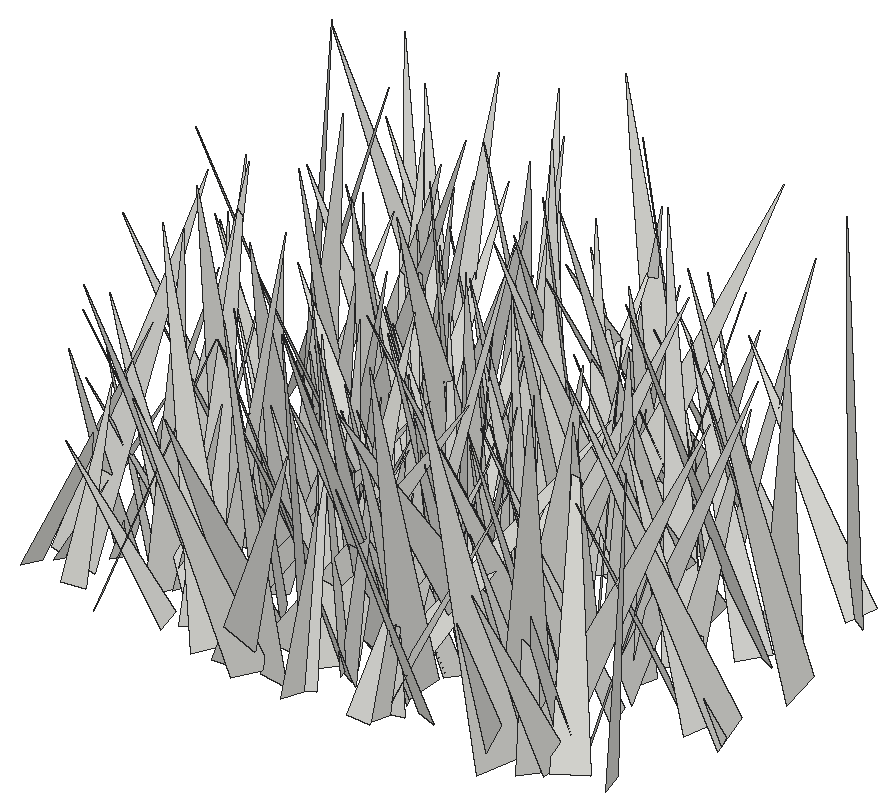
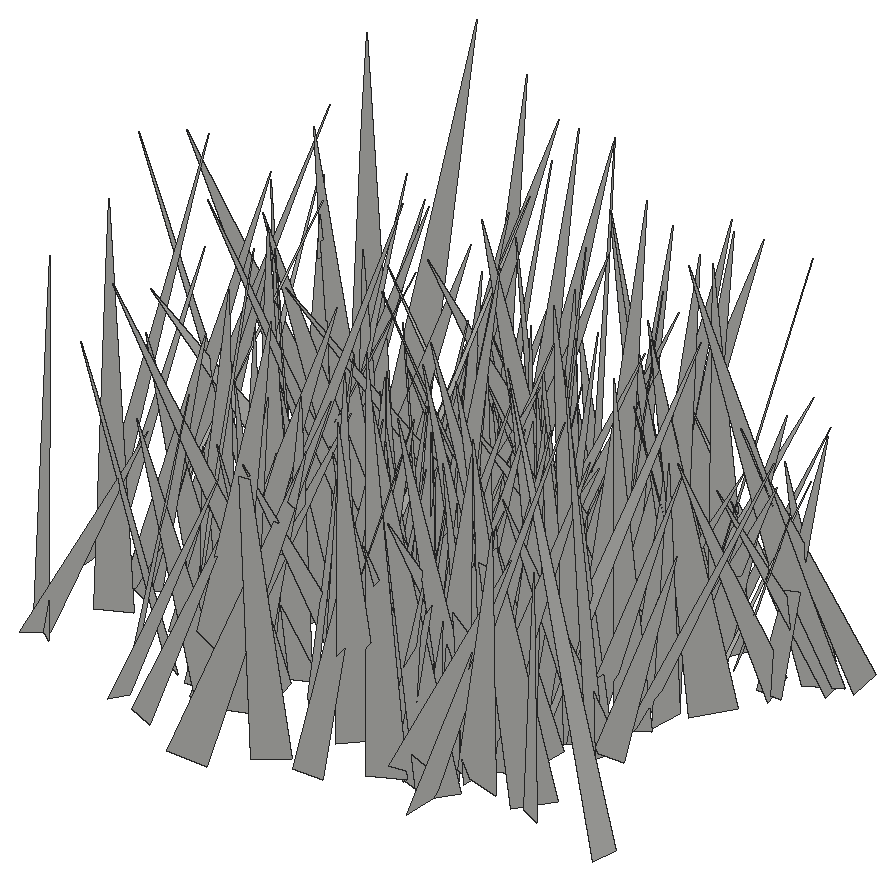
# SketchUp Ruby script. Lengths in inches.
U = 1.inch
M = Sketchup.active_model
def pt(a) = Geom::Point3d.new(a.map { |v| v * U })
def face(e, loops, mat)
  f = e.add_face(loops[0].map { |a| pt(a) })
  loops[1..].each { |l| e.add_face(l.map { |a| pt(a) }).erase! }
  f.material = f.back_material = mat if mat
  f
end
# faces: each face lists its corners as indices into pts; further lists are holes
def faces(e, pts, list, mat = nil) = list.each { |f| face(e, (f[0].is_a?(Array) ? f : [f]).map { |l| l.map { |i| pts[i] } }, mat) }
# xy, xz, yz: faces in a plane at the given z, y or x. An outline is a flat list of corners, or four numbers for a rectangle; further outlines are holes
def ring(l) = l.size == 4 ? [[l[0], l[1]], [l[2], l[1]], [l[2], l[3]], [l[0], l[3]]] : l.each_slice(2).to_a
def flat(e, list, mat, &to3) = list.each { |f| face(e, (f[0].is_a?(Array) ? f : [f]).map { |l| ring(l).map { |u, v| to3.(u, v) } }, mat) }
def xy(e, z, list, mat = nil) = flat(e, list, mat) { |x, y| [x, y, z] }
def xz(e, y, list, mat = nil) = flat(e, list, mat) { |x, z| [x, y, z] }
def yz(e, x, list, mat = nil) = flat(e, list, mat) { |y, z| [x, y, z] }
def lines(e, pts, list) = list.each { |a, b| e.add_line(pt(pts[a]), pt(pts[b])) }
# prism: a flat outline (further loops are holes) pulled along v
def prism(e, loops, v, mat = nil)
  f = face(e, loops, mat); d = Geom::Vector3d.new(v.map { |x| x * U })
  f.pushpull(f.normal.samedirection?(d) ? d.length : -d.length)
end
def box(e, o, s, mat = nil) = prism(e, [[o, [o[0] + s[0], o[1], o[2]], [o[0] + s[0], o[1] + s[1], o[2]], [o[0], o[1] + s[1], o[2]]]], [0, 0, s[2]], mat)
def at(x, y, z, deg = 0) = Geom::Transformation.translation(pt([x, y, z])) * Geom::Transformation.rotation(ORIGIN, Z_AXIS, deg.degrees)
def axes(o, x, y, z) = Geom::Transformation.new([*x, 0, *y, 0, *z, 0, *pt(o).to_a, 1])
def part(name) = M.definitions.add(name)
# library, detail: a bought-in or finely detailed component or shape, given as its bounding box
def library(name, o, s) = part(name).tap { |d| box(d.entities, o, s) }
def detail(e, o, s) = box(e.add_group.entities, o, s)
def put(e, d, t, mat = nil) = e.add_instance(d, t).tap { |i| i.material = mat if mat }
def group(e, t, mat = nil) = e.add_group.tap { |g| g.transformation = t; g.material = mat if mat }.entities
root = M.entities
c1 = part("fur_instance\#9")
p = [[0.8125,0,1.79],[0.67,-0.02,1.48],[0,-0.11,0],[0,0.11,0]]
faces(c1.entities,p,[[0,1,2,3]])
put(root,c1,axes([490.59,5.4,-21.86],[2.87814,-5.28951,1.31735],[-4.95416,-3.15966,-1.86304],[-2.27391,0.18887,5.72641]))
put(root,c1,axes([500.76,5.73,-21.86],[6.46231,-4.31648,2.52967],[-3.92803,-6.93665,-1.8017],[-3.09867,-0.20881,7.55958]))
put(root,c1,axes([489.84,5.36,-21.86],[2.89446,-5.47209,0.08006],[-5.31049,-2.7865,1.53693],[1.32243,0.78724,5.99662]))
put(root,c1,axes([500.48,6.03,-21.86],[4.1039,-1.37964,0.4984],[-1.03776,-3.77714,-1.91052],[-1.03675,-1.68037,3.88527]))
put(root,c1,axes([489.15,7.79,-21.86],[5.11337,-4.37567,0.02712],[-4.08728,-4.79107,-2.37351],[-1.56248,-1.78687,6.29758]))
put(root,c1,axes([502.23,6.75,-21.86],[4.14247,-2.36814,0.94959],[-1.79033,-3.98803,-2.13546],[-1.81783,-1.46881,4.26707]))
put(root,c1,axes([492.5625,5.1,-21.86],[3.76138,-1.24538,0.93866],[-1.27843,-3.86595,-0.00634],[-0.89313,0.28885,3.96218]))
put(root,c1,axes([486.36,6.41,-21.86],[-3.93279,-0.23592,0.50656],[-0.05149,3.7386,1.34138],[0.55643,-1.32147,3.70448]))
put(root,c1,axes([491.49,5.47,-21.86],[1.25077,5.74635,3.18749],[6.40163,-1.79789,0.7292],[-1.48314,-2.91412,5.83551]))
put(root,c1,axes([491.71,6.95,-21.86],[6.5233,2.37968,3.04495],[3.30026,-6.53866,-1.96019],[-2.01069,-3.01183,6.66138]))
put(root,c1,axes([495.69,7.7,-21.86],[7.48346,-2.4752,1.75576],[-1.96533,-7.51292,-2.21472],[-2.31232,-1.62508,7.56464]))
put(root,c1,axes([496.91,6.61,-21.86],[-1.89303,-4.40404,0.51291],[-4.43222,1.86471,-0.34716],[-0.11875,0.60786,4.78107]))
put(root,c1,axes([495.44,7.87,-21.86],[-5.97447,-2.65496,2.2585],[-2.10106,6.3191,1.8704],[2.78122,-0.92951,6.26456]))
put(root,c1,axes([499.77,8.2,-21.86],[5.80631,-5.6916,0.53269],[-5.68589,-5.82856,-0.29992],[-0.59055,0.15799,8.12513]))
put(root,c1,axes([495.26,5.15,-21.86],[-0.85161,3.55792,0.87868],[3.50079,1.05663,-0.88551],[1.08413,-0.61714,3.54963]))
put(root,c1,axes([495.77,5.74,-21.86],[3.9323,-0.29865,1.47953],[-0.48436,-4.16008,0.44758],[-1.42954,0.58799,3.91814]))
put(root,c1,axes([488.64,5.97,-21.86],[5.34271,-3.44394,4.19103],[-3.85612,-6.54857,-0.46545],[-3.8152,1.796,6.33945]))
put(root,c1,axes([492.67,5.54,-21.86],[-2.63101,2.88231,1.12737],[2.88894,2.81797,-0.46255],[1.11028,-0.50218,3.87505]))
put(root,c1,axes([493.65,9.14,-21.86],[-1.56855,-7.63886,0.47282],[-7.63369,1.59619,0.46371],[0.55001,0.36889,7.78444]))
put(root,c1,axes([493.09,9.02,-21.86],[-1.24529,-7.71146,0.7872],[-7.61167,1.36728,1.35282],[1.46589,0.54863,7.69333]))
put(root,c1,axes([495.97,6.11,-21.86],[-0.42673,3.51272,1.26133],[3.73148,0.37463,0.21911],[-0.0791,-1.27778,3.53176]))
put(root,c1,axes([485.99,8.94,-21.86],[-5.87667,-3.9224,1.1719],[-3.54254,5.90008,1.98324],[2.05159,-1.04767,6.78139]))
put(root,c1,axes([496.43,11.28,-21.86],[6.48177,-5.01878,0.45242],[-4.24735,-5.8379,-3.90962],[-2.71162,-2.85253,7.2053]))
put(root,c1,axes([482.5,6.33,-21.86],[1.50954,-3.07856,1.78204],[-3.55315,-1.39659,0.59714],[-0.16832,1.87187,3.37633]))
put(root,c1,axes([495.36,6.375,-21.86],[4.26257,2.91433,0.00484],[2.86478,-4.18851,-0.95515],[0.53516,-0.79116,5.0745]))
put(root,c1,axes([493.22,7.15,-21.86],[-4.07281,-4.5818,0.7427],[-4.55178,3.7491,-1.83244],[-0.90871,1.75604,5.85003]))
put(root,c1,axes([502.5,7.23,-21.86],[-2.82559,-5.19892,1.36333],[-5.31081,2.46391,-1.61114],[-0.82624,1.9421,5.69358]))
put(root,c1,axes([493.16,7.29,-21.86],[-2.2184,-4.85625,2.50772],[-5.03427,2.86928,1.10295],[2.1279,1.72546,5.22379]))
put(root,c1,axes([483.85,5.87,-21.86],[4.67763,2.46387,0.32375],[2.42875,-4.67875,0.51598],[-0.52599,0.30722,5.26162]))
put(root,c1,axes([488.33,6.51,-21.86],[3.51282,6.48869,2.15536],[6.79895,-3.57131,-0.32959],[-0.72316,-2.057,7.37118]))
put(root,c1,axes([494.02,9.8,-21.86],[0.91658,-6.09487,0.23316],[-5.96683,-0.94489,-1.24341],[-1.26442,0.04079,6.03668]))
put(root,c1,axes([504.33,6.97,-21.86],[-4.83531,-1.63891,2.39644],[-2.01972,5.24312,-0.48946],[2.08559,1.27782,5.08199]))
put(root,c1,axes([485.08,7.92,-21.86],[-5.61419,2.77509,3.47904],[3.15086,6.4338,-0.04739],[3.14276,-1.49299,6.26243]))
put(root,c1,axes([486.97,8.74,-21.86],[-3.76268,-4.24685,0.11424],[-4.17448,3.66755,-1.15295],[-0.78896,0.84846,5.55555]))
put(root,c1,axes([480.48,6.67,-21.86],[5.14686,-0.10254,0.48257],[-0.21946,-5.00543,1.27711],[-0.44184,1.29176,4.98695]))
put(root,c1,axes([482.52,9.11,-21.86],[-0.08561,-4.51883,0.61864],[-4.55746,0.06047,-0.18896],[-0.17898,0.62161,4.51569]))
put(root,c1,axes([492.46,7.47,-21.86],[-4.38445,3.57185,1.79964],[3.76738,4.58485,0.07863],[1.34299,-1.20052,5.65467]))
put(root,c1,axes([501.79,5.78,-21.86],[-6.16922,0.32467,1.04524],[-0.06119,5.87189,-2.18505],[1.09279,2.16166,5.77844]))
put(root,c1,axes([492.85,7.61,-21.86],[-6.07164,-2.28107,2.04855],[-2.55827,6.27412,-0.5961],[1.68971,1.3026,6.45854]))
put(root,c1,axes([491.02,9.64,-21.86],[-1.13114,-4.608,0.05517],[-4.59723,1.12439,-0.34274],[-0.31976,0.13515,4.73241]))
put(root,c1,axes([490.4,7.86,-21.86],[4.34126,2.62004,0.01209],[2.52851,-4.18338,-1.34808],[0.68659,-1.1602,4.88813]))
put(root,c1,axes([490.38,7.3125,-21.86],[4.70359,-4.43483,0.77561],[-4.1988,-3.91632,3.07011],[1.62462,2.71804,5.6891]))
put(root,c1,axes([502.88,6.61,-21.86],[-3.10471,5.12305,0.88051],[5.18598,3.12286,0.11631],[0.35573,-0.81381,5.98927]))
put(root,c1,axes([489.07,9.04,-21.86],[-4.89402,-3.33819,1.83703],[-3.30827,5.20635,0.64726],[1.89038,0.46913,5.88863]))
put(root,c1,axes([500.16,10.02,-21.86],[-3.94207,-4.94022,1.13908],[-4.81769,4.09962,1.10733],[1.57897,0.1748,6.2225]))
put(root,c1,axes([485.38,8.5,-21.86],[3.78435,-1.32179,0.68035],[-1.35222,-3.83372,0.07338],[-0.61764,0.29457,4.00787]))
put(root,c1,axes([492.36,7.69,-21.86],[-1.02594,6.32348,2.52203],[6.58274,1.57191,-1.26344],[1.73626,-2.22313,6.28034]))
put(root,c1,axes([491.15,9.28,-21.86],[1.24719,-3.91493,0.4967],[-3.8954,-1.13791,0.81231],[0.63182,0.71228,4.02769]))
put(root,c1,axes([492.39,9.25,-21.86],[-1.33091,-4.34516,1.37723],[-4.35803,1.6335,0.94222],[1.33595,0.99989,4.44566]))
put(root,c1,axes([485.41,8.57,-21.86],[0.69074,-4.72184,2.34998],[-4.89788,-1.45354,-1.48096],[-1.95676,1.97148,4.53648]))
put(root,c1,axes([481.08,7.53,-21.86],[4.0967,-0.1052,0.02727],[-0.10864,-3.93802,1.12914],[0.00278,1.12946,3.93942]))
put(root,c1,axes([486.375,8.03,-21.86],[-2.33068,3.85921,0.35584],[3.66264,2.05758,1.6744],[-1.26695,-1.15111,4.18592]))
put(root,c1,axes([481.46,7.63,-21.86],[0.24663,7.62872,2.41582],[7.70784,0.42293,-2.12242],[2.15005,-2.39126,7.33168]))
put(root,c1,axes([496.5,9.66,-21.86],[-2.38494,-6.16406,1.52656],[-6.35023,2.30898,-0.59758],[-0.0234,1.63919,6.58229]))
put(root,c1,axes([500.99,7.71,-21.86],[5.79439,-3.93356,1.43708],[-4.17619,-5.2444,2.48372],[0.31237,2.85246,6.54821]))
put(root,c1,axes([484.71,7.97,-21.86],[-3.84784,-1.19504,0.32807],[-1.23606,3.62421,-1.29571],[-0.08892,1.33363,3.81512]))
put(root,c1,axes([498.37,9.9,-21.86],[-3.36385,-0.86607,1.07357],[-0.51946,3.41676,1.12873],[1.27781,-0.89095,3.28504]))
put(root,c1,axes([495.2,9.57,-21.86],[-3.34237,-3.67886,0.49489],[-3.71061,3.29315,-0.58039],[-0.10119,0.75599,4.93646]))
put(root,c1,axes([484.01,10.37,-21.86],[-3.17916,-2.57933,0.00353],[-2.53731,3.12837,0.73174],[0.46373,-0.56605,4.02798]))
put(root,c1,axes([497.12,9.2,-21.86],[-3.3946,-3.12525,1.18102],[-3.29173,3.41661,-0.4203],[0.5714,1.11577,4.59499]))
put(root,c1,axes([498.01,11.3,-21.86],[2.24091,-5.47361,0.67385],[-5.23088,-2.33999,-1.61199],[-1.7471,-0.01469,5.69066]))
put(root,c1,axes([490.29,8.67,-21.86],[4.49912,0.07902,0.02983],[0.07502,-4.46879,0.52292],[-0.03881,0.52233,4.46932]))
put(root,c1,axes([490.03,10.12,-21.86],[1.8485,-3.49978,1.33816],[-3.45042,-2.17169,-0.91344],[-1.46071,0.70098,3.8511]))
put(root,c1,axes([502.19,12.9,-21.86],[-3.50557,-5.51536,0.11612],[-4.95597,3.20905,2.80393],[2.42302,-1.41579,5.90306]))
put(root,c1,axes([498.3,10.3125,-21.86],[2.2039,-6.87435,1.74953],[-7.02125,-1.85328,1.56272],[1.00974,2.1174,7.04782]))
put(root,c1,axes([495.91,9.36,-21.86],[-0.77186,4.35622,1.72795],[4.2436,-0.09339,2.13104],[-1.98854,-1.8902,3.87699]))
put(root,c1,axes([505.26,11.92,-21.86],[-7.42684,-1.75978,1.28146],[-1.36577,7.3143,2.12899],[1.69519,-1.81689,7.32954]))
put(root,c1,axes([501.73,10.57,-21.86],[-5.35424,-1.86738,0.02315],[-1.86377,5.3475,0.29345],[0.11847,-0.26947,5.66294]))
put(root,c1,axes([487.11,12.33,-21.86],[7.37439,-3.31849,1.28024],[-2.90244,-7.31769,-2.24953],[-2.05603,-1.57231,7.76747]))
put(root,c1,axes([494.46,7.55,-21.86],[0.90469,6.24799,0.05202],[5.52251,-0.775,-2.9597],[2.92267,-0.46962,5.57638]))
put(root,c1,axes([487.34,6.8,-21.86],[-7.34828,2.49323,1.09592],[2.03506,7.1224,-2.5582],[1.80991,2.11416,7.32591]))
put(root,c1,axes([489.42,10.99,-21.86],[2.10827,-4.41232,0.88185],[-4.4927,-2.11805,0.1432],[-0.24874,0.85808,4.88803]))
put(root,c1,axes([493.11,9.65,-21.86],[1.63148,3.88333,0.8996],[3.80186,-1.22375,-1.61232],[1.19808,-1.40479,3.89132]))
put(root,c1,axes([499.21,11.93,-21.86],[1.92624,-6.27783,0.49509],[-6.26935,-1.863,0.76884],[0.59288,0.69623,6.52153]))
put(root,c1,axes([493.19,12.73,-21.86],[5.45875,-2.61976,0.1584],[-2.41646,-5.15945,-2.05595],[-1.02417,-1.78972,5.6951]))
put(root,c1,axes([496.29,13.07,-21.86],[-5.79035,-4.99721,0.36352],[-4.82955,5.71454,1.62848],[1.33407,-1.00217,7.47317]))
put(root,c1,axes([485.17,11.72,-21.86],[2.46891,-7.20313,1.70316],[-7.36136,-2.57683,-0.22704],[-0.77207,1.53499,7.61111]))
put(root,c1,axes([484.84,9.4,-21.86],[3.62084,3.81527,1.03017],[3.87963,-3.69771,0.05854],[-0.75237,-0.70613,5.25959]))
put(root,c1,axes([497.61,10.52,-21.86],[3.73995,-4.97965,1.07609],[-4.97131,-3.27521,2.12161],[1.114,2.10195,5.85517]))
put(root,c1,axes([482.49,8.72,-21.86],[4.99403,0.89918,1.35491],[0.3935,-4.91429,1.81096],[-1.5778,1.62046,4.74018]))
put(root,c1,axes([487.35,9.11,-21.86],[4.61387,-2.10989,0.31356],[-1.93342,-3.82099,2.73855],[0.90102,2.60502,4.2708]))
put(root,c1,axes([488.07,10.05,-21.86],[3.36091,-1.13304,0.9234],[-1.35023,-3.29337,0.87337],[-0.55977,1.1411,3.43755]))
put(root,c1,axes([486.82,11.87,-21.86],[-2.52034,-4.28654,0.32351],[-4.12689,2.30776,-1.57296],[-1.20326,1.06349,4.71724]))
put(root,c1,axes([505.29,11.7,-21.86],[-6.30191,-3.29477,0.26908],[-3.30318,6.25333,-0.79169],[-0.13009,0.82599,7.06702]))
put(root,c1,axes([490.69,11.97,-21.86],[-4.19066,-2.50752,1.09961],[-2.47633,4.32875,0.43379],[1.16817,0.18082,4.86427]))
put(root,c1,axes([504.32,11.56,-21.86],[-4.9541,1.83691,1.27432],[2.05779,4.95762,0.85363],[0.87385,-1.26054,5.21428]))
put(root,c1,axes([494.57,7.87,-21.86],[3.62911,6.60842,0.2466],[6.35712,-3.56375,1.94657],[-1.82181,0.72867,7.28371]))
put(root,c1,axes([483.18,11.19,-21.86],[5.12672,-4.5376,2.59386],[-5.0883,-5.16347,1.02416],[-1.19461,2.5199,6.76936]))
put(root,c1,axes([490.99,13.09,-21.86],[-3.68425,-5.36529,0.32526],[-5.32374,3.58793,-1.11818],[-0.74155,0.8979,6.41168]))
put(root,c1,axes([495.29,12.36,-21.86],[-1.22069,-3.41408,1.05948],[-3.55821,1.26785,-0.01408],[0.34288,1.00256,3.62571]))
put(root,c1,axes([491.7,12.59,-21.86],[-3.20699,2.34244,2.63387],[2.95903,3.72406,0.29089],[1.91533,-1.83124,3.96071]))
put(root,c1,axes([500.59,12.28,-21.86],[4.54413,5.8348,1.67226],[5.93472,-3.83302,-2.75273],[1.27295,-2.95864,6.86415]))
put(root,c1,axes([495.35,12.3,-21.86],[-0.92871,-3.83483,1.6083],[-4.04735,1.2119,0.55253],[0.95473,1.40727,3.90681]))
put(root,c1,axes([488.81,12.55,-21.86],[0.02782,-4.7345,1.86898],[-5.06027,0.17616,0.52158],[0.54982,1.86087,4.70577]))
put(root,c1,axes([501,12.83,-21.86],[3.6892,-1.49713,1.29137],[-1.47127,-3.90506,-0.32413],[-1.32076,0.16824,3.96818]))
put(root,c1,axes([484.48,13.72,-21.86],[2.19919,-5.46865,1.19281],[-5.58851,-2.07385,0.79564],[0.31218,1.39943,5.84033]))
put(root,c1,axes([484.4375,13.72,-21.86],[-5.87087,-0.65311,0.1721],[-0.62527,5.82501,0.77566],[0.25536,-0.75237,5.85594]))
put(root,c1,axes([496.43,11.58,-21.86],[3.12045,6.97557,0.92804],[6.87353,-2.80376,-2.03727],[1.5081,-1.6545,7.36514]))
put(root,c1,axes([502.36,8.17,-21.86],[5.94606,5.36025,0.59468],[4.2161,-5.17199,4.4628],[-3.36309,2.9933,6.64615]))
put(root,c1,axes([484.04,12.55,-21.86],[-5.13165,1.21269,1.54361],[1.09048,5.35359,-0.58061],[1.63224,0.23592,5.24093]))
put(root,c1,axes([498.89,14.3,-21.86],[2.3512,-5.85332,1.44977],[-6.03015,-2.28819,0.5412],[-0.02311,1.54732,6.28463]))
put(root,c1,axes([492.91,13.8,-21.86],[4.61711,2.95667,1.94744],[3.35791,-4.67134,-0.86895],[-1.12198,-1.8135,5.41336]))
put(root,c1,axes([491.25,12.68,-21.86],[-3.06534,4.86368,0.18481],[4.51167,2.75744,2.26433],[-1.82603,-1.35165,5.28436]))
put(root,c1,axes([493.16,14,-21.86],[4.30698,0.82715,0.77594],[0.97071,-4.26434,-0.84231],[-0.5865,-0.98365,4.30404]))
put(root,c1,axes([493.02,13.8125,-21.86],[-2.4507,-4.58404,1.24543],[-4.71435,2.17524,-1.27033],[-0.58261,1.68089,5.0404]))
put(root,c1,axes([498.07,14,-21.86],[4.89735,3.35239,2.18214],[3.80193,-4.97328,-0.89225],[-1.24321,-2.00306,5.86741]))
put(root,c1,axes([496.82,11.96,-21.86],[1.00631,5.78428,1.17144],[5.41169,-1.37849,2.15781],[-2.35451,-0.6962,5.46025]))
put(root,c1,axes([487.01,15.53,-21.86],[-4.99858,-6.00178,0.67378],[-6.03784,4.94565,-0.739],[-0.1407,0.9901,7.77567]))
put(root,c1,axes([498.68,16.22,-21.86],[-7.7703,-1.5883,1.42664],[-1.2052,7.70803,2.01725],[1.76224,-1.7318,7.67014]))
put(root,c1,axes([485.99,14.05,-21.86],[-5.48132,1.03762,0.48302],[1.07413,5.47965,0.41785],[0.39525,-0.50168,5.563]))
put(root,c1,axes([486.99,14.62,-21.86],[5.5976,-0.64404,1.05715],[-0.59203,-5.69245,-0.3332],[-1.08713,-0.21617,5.62467]))
put(root,c1,axes([485.53,15.73,-21.86],[0.81031,-5.69395,0.84212],[-5.55553,-0.55126,1.61834],[1.50543,1.03047,5.51893]))
put(root,c1,axes([502.82,16.57,-21.86],[-3.23676,-6.95107,0.75182],[-6.9834,3.25434,0.02332],[0.33861,0.67166,7.66769]))
put(root,c1,axes([485.76,15.4,-21.86],[-0.85908,-3.57953,0.71794],[-3.54097,0.99653,0.73143],[0.88884,0.51028,3.60778]))
put(root,c1,axes([491.31,14.39,-21.86],[-4.79619,2.23097,0.90337],[2.34699,4.78153,0.65218],[0.53379,-0.97799,5.24932]))
put(root,c1,axes([505.27,15.57,-21.86],[-7.82049,-1.65264,1.82204],[-1.48703,8.01344,0.88582],[1.95953,-0.51451,7.94397]))
put(root,c1,axes([486.48,16.1,-21.86],[6.50516,0.09741,3.11354],[0.81371,-7.01185,-1.48071],[-3.00691,-1.68675,6.33514]))
put(root,c1,axes([496.86,14.3125,-21.86],[3.28542,-2.52777,1.83261],[-2.97263,-3.34603,0.71392],[-0.95477,1.71946,4.08337]))
put(root,c1,axes([485.35,15.01,-21.86],[6.93717,-2.75986,2.51351],[-2.97128,-7.29338,0.19237],[-2.25967,1.11744,7.46352]))
put(root,c1,axes([494.14,15.56,-21.86],[1.8151,-3.86013,1.55176],[-3.9232,-2.15155,-0.76319],[-1.38458,1.03602,4.19675]))
put(root,c1,axes([492.125,13.58,-21.86],[3.50829,2.33455,0.59392],[2.17247,-3.51961,1.00185],[-1.04078,0.52272,4.09323]))
put(root,c1,axes([492.63,13.39,-21.86],[-4.5545,1.12209,0.15618],[1.0267,4.36161,-1.39615],[0.47894,1.3207,4.4781]))
put(root,c1,axes([489.69,18.05,-21.86],[7.10031,-2.91459,1.55919],[-2.29482,-7.00551,-2.64516],[-2.37902,-1.94118,7.20502]))
put(root,c1,axes([492.23,14.33,-21.86],[-4.76219,-1.42096,1.84075],[-1.91994,4.76946,-1.2853],[1.31199,1.82182,4.80058]))
put(root,c1,axes([504.17,16.65,-21.86],[-3.86878,-4.9807,0.99535],[-5.05831,3.89149,-0.18804],[0.45997,0.9025,6.30392]))
put(root,c1,axes([500.94,15.1875,-21.86],[4.04203,-2.33275,1.48439],[-2.65208,-4.01454,0.91276],[-0.78205,1.55722,4.57675]))
put(root,c1,axes([491.38,15.71,-21.86],[-3.99444,1.28958,0.25526],[1.31279,3.95594,0.55757],[0.06915,-0.60932,4.16025]))
put(root,c1,axes([483.97,15.61,-21.86],[-2.38269,3.95567,1.05235],[4.03891,2.07425,1.34786],[-0.66484,-1.57548,4.41677]))
put(root,c1,axes([500.03,17.9375,-21.86],[3.38324,-1.277,0.34003],[-0.90165,-2.91389,-1.97203],[-0.96612,-1.75247,3.03119]))
put(root,c1,axes([490.88,15.92,-21.86],[-5.61783,-2.93903,2.21928],[-3.25584,5.85535,-0.48739],[1.72124,1.48327,6.32142]))
put(root,c1,axes([490.4,17.31,-21.86],[1.13187,-5.42392,1.09616],[-5.52646,-1.05128,0.50466],[0.2806,1.17367,5.51773]))
put(root,c1,axes([490.66,15.08,-21.86],[-5.41908,-0.82486,1.13145],[-1.12996,5.24719,-1.58656],[0.82691,1.76453,5.24687]))
put(root,c1,axes([498.25,16.33,-21.86],[-3.46887,0.5768,0.94943],[0.60796,3.5911,0.03958],[0.92978,-0.19616,3.51628]))
put(root,c1,axes([502.57,18.03,-21.86],[1.17808,-6.7396,1.1437],[-6.76699,-0.98532,1.16408],[0.96855,1.31342,6.74203]))
put(root,c1,axes([502.72,16.34,-21.86],[-3.89894,3.87426,1.21258],[4.05705,3.77806,0.97396],[0.14352,-1.54866,5.40953]))
put(root,c1,axes([501.22,14.56,-21.86],[-7.08431,2.74004,0.68893],[2.60293,7.0529,-1.28499],[1.09872,0.95845,7.48626]))
put(root,c1,axes([488.25,16.15,-21.86],[6.43486,-0.85229,1.84553],[-1.08084,-6.62327,0.70985],[-1.72168,0.97247,6.45212]))
put(root,c1,axes([489.56,16.13,-21.86],[-3.69275,-0.52533,1.17947],[-0.76187,3.77166,-0.70545],[1.04243,0.89562,3.66261]))
put(root,c1,axes([485.71,18.33,-21.86],[3.36896,-5.0045,1.18358],[-5.04079,-3.49374,-0.42432],[-1.01802,0.73793,6.01788]))
put(root,c1,axes([484.15,15.625,-21.86],[4.14579,-2.60609,2.17076],[-3.31381,-3.84297,1.71517],[-0.72292,2.67047,4.58667]))
put(root,c1,axes([487.96,17.79,-21.86],[-2.42816,-5.42807,1.43938],[-5.61543,2.33238,-0.67728],[-0.05217,1.5899,5.90772]))
put(root,c1,axes([484.4,15.77,-21.86],[-7.10447,-2.39928,3.44832],[-3.25719,7.42464,-1.54476],[2.65295,2.69055,7.33783]))
put(root,c1,axes([488.5,16.16,-21.86],[-4.11869,2.39634,0.55767],[2.352,4.15398,-0.47915],[0.72219,0.13795,4.74094]))
put(root,c1,axes([485.39,17.13,-21.86],[7.44021,-1.05618,0.97458],[-1.13327,-7.472,0.55406],[-0.88376,0.68976,7.49435]))
put(root,c1,axes([498.02,18.29,-21.86],[-1.13695,-6.80591,1.9758],[-6.92615,0.64332,-1.76957],[-1.50086,2.18691,6.66945]))
put(root,c1,axes([490.05,16.61,-21.86],[-3.61656,3.24074,0.55892],[3.26072,3.64166,-0.01623],[0.42715,-0.36083,4.85609]))
put(root,c1,axes([486.79,19.02,-21.86],[-5.48359,2.23586,1.70204],[2.68404,5.27249,1.72124],[0.83185,-2.27324,5.66623]))
put(root,c1,axes([497.78,18.99,-21.86],[2.79472,-2.37927,0.19168],[-2.37504,-2.80125,-0.14262],[-0.23842,0.01542,3.66757]))
put(root,c1,axes([490.98,19.09,-21.86],[-4.40075,-1.21691,1.44212],[-0.98766,4.60363,0.87078],[1.60783,-0.50284,4.4821]))
put(root,c1,axes([487.38,16.93,-21.86],[-1.64071,6.20292,1.41522],[6.35653,1.66047,0.09149],[0.27128,-1.39198,6.41559]))
put(root,c1,axes([483.9,19.56,-21.86],[3.71453,-6.09838,0.78607],[-6.05056,-3.46164,1.73599],[1.09493,1.55972,6.92635]))
put(root,c1,axes([493.59,19.07,-21.86],[-4.35453,-4.53446,2.05004],[-4.74623,4.60317,0.10013],[1.49574,1.4055,6.28595]))
put(root,c1,axes([495.45,17.65,-21.86],[-5.08391,3.17186,1.29588],[3.17676,5.23223,-0.34381],[1.28383,-0.38638,5.98237]))
put(root,c1,axes([494.31,17.31,-21.86],[-6.74391,-2.32387,0.77011],[-2.44649,6.31426,-2.37034],[-0.09,2.49068,6.72772]))
put(root,c1,axes([498.99,18.64,-21.86],[-6.4254,-4.61842,2.37343],[-5.01235,6.50279,-0.91585],[1.35622,2.15235,7.85982]))
put(root,c1,axes([488.64,15.45,-21.86],[-4.56686,4.07542,0.09193],[3.68922,4.19072,-2.51023],[1.73411,1.8173,5.58247]))
put(root,c1,axes([490.34,17.2,-21.86],[-2.89622,3.26829,0.45856],[3.08153,2.89643,-1.18106],[1.18158,0.4572,4.20415]))
put(root,c1,axes([493.62,16.54,-21.86],[-1.51981,5.35977,0.02073],[5.22969,1.48762,-1.21441],[1.17387,0.31183,5.43711]))
put(root,c1,axes([492.98,18.14,-21.86],[-0.82841,6.75025,1.93378],[7.00258,0.65031,0.72978],[-0.51887,-2.00072,6.76162]))
put(root,c1,axes([486.96,20.23,-21.86],[4.55576,-0.64185,1.19418],[-0.37344,-4.61891,-1.05794],[-1.3033,-0.92017,4.47746]))
put(root,c1,axes([496.81,18.27,-21.86],[-1.73609,5.26171,0.91511],[5.1615,1.40586,1.70864],[-1.37182,-1.3693,5.27069]))
put(root,c1,axes([486.53,19.33,-21.86],[5.43956,-0.0104,1.6458],[0.01524,-5.68242,-0.08629],[-1.64576,-0.087,5.43889]))
put(root,c1,axes([496.87,20.95,-21.86],[-2.5051,-3.46967,0.23869],[-3.39401,2.50314,0.76559],[0.75915,-0.25846,4.21047]))
put(root,c1,axes([496.4,21.21,-21.86],[-1.56968,-5.60909,0.11931],[-5.50885,1.51747,-1.1357],[-1.06238,0.41882,5.71278]))
put(root,c1,axes([480.02,20.77,-21.86],[8.03575,1.73258,0.69022],[1.85682,-7.7181,-2.24381],[-0.17451,-2.34107,7.90825]))
put(root,c1,axes([488.78,18.02,-21.86],[-5.17368,4.83178,0.63052],[4.85594,5.1888,0.08232],[0.40437,-0.49072,7.07858]))
put(root,c1,axes([494.89,17.83,-21.86],[1.48421,7.77893,1.22221],[7.56365,-1.06243,-2.42301],[2.19017,-1.60247,7.53948]))
put(root,c1,axes([486.64,21.08,-21.86],[3.61715,-5.66391,0.01487],[-5.50634,-3.51236,1.58351],[1.3268,0.86448,6.53117]))
put(root,c1,axes([495.34,20.77,-21.86],[2.16413,-4.87719,1.14426],[-4.95965,-2.26151,-0.2591],[-0.70577,0.93721,5.32947]))
put(root,c1,axes([494.88,18.88,-21.86],[4.75143,0.92242,1.33841],[0.70934,-4.89704,0.85681],[-1.46255,0.62163,4.7637]))
put(root,c1,axes([488.79,21.14,-21.86],[1.17018,-6.95871,1.51726],[-7.0392,-0.89595,1.31981],[1.08411,1.69372,6.93189]))
put(root,c1,axes([491.93,17.23,-21.86],[-6.30964,2.41528,1.06239],[1.96226,6.1361,-2.29599],[1.76402,1.81341,6.35402]))
put(root,c1,axes([488.56,20.72,-21.86],[-2.7828,-3.97435,1.2381],[-4.07565,2.90431,0.16237],[0.84701,0.91751,4.84903]))
put(root,c1,axes([487.83,18.18,-21.86],[0.08321,7.29137,1.2347],[7.39423,-0.10178,0.10277],[-0.11831,-1.23331,7.29112]))
put(root,c1,axes([489.28,20.29,-21.86],[-3.6032,0.74818,1.09352],[0.87855,3.72087,0.34907],[0.99182,-0.57787,3.66346]))
put(root,c1,axes([483.52,20.24,-21.86],[-1.7362,-3.80786,1.79903],[-4.13168,1.91701,0.07019],[0.81577,1.60498,4.18441]))
put(root,c1,axes([490.91,22.53,-21.86],[-0.42981,-6.03201,0.26249],[-6.01913,0.44871,0.45551],[0.47339,0.22867,6.03012]))
put(root,c1,axes([503.69,20.7,-21.86],[-4.58774,2.19144,0.09862],[2.15217,4.45217,1.18567],[-0.42461,-1.11142,4.94408]))
put(root,c1,axes([498.83,19.72,-21.86],[3.4607,5.10853,1.2476],[5.25066,-3.43918,-0.48234],[-0.29016,-1.30574,6.15149]))
put(root,c1,axes([499.48,21.05,-21.86],[-4.91949,-2.25789,1.34677],[-2.33985,5.06309,-0.05864],[1.19873,0.61667,5.41258]))
put(root,c1,axes([503.7,20.39,-21.86],[-3.98091,-5.38333,3.048],[-6.04161,4.16252,-0.53901],[1.33021,2.79489,6.67363]))
put(root,c1,axes([496.07,20.95,-21.86],[3.98681,-3.04122,0.56389],[-3.08769,-3.85909,1.01744],[0.18196,1.14894,4.91004]))
put(root,c1,axes([486.72,21.9,-21.86],[-7.8071,-1.03462,1.04066],[-0.93299,7.84786,0.80297],[1.13267,-0.66693,7.83431]))
put(root,c1,axes([494.61,24.21,-21.86],[3.27442,-5.47757,0.11686],[-5.10679,-3.10069,-2.24625],[-1.98447,-1.05885,5.97327]))
put(root,c1,axes([496.77,20.26,-21.86],[-3.07753,7.46975,2.03134],[7.70521,2.74591,1.57617],[-0.74375,-2.46119,7.92363]))
put(root,c1,axes([490.92,19.82,-21.86],[-4.66477,5.25581,1.41142],[5.28211,4.8201,-0.49149],[1.30953,-0.72026,7.01013]))
put(root,c1,axes([488.21,20.91,-21.86],[-1.67581,5.69721,1.32161],[5.39716,0.9769,2.63242],[-2.25291,-1.89755,5.32325]))
put(root,c1,axes([498.88,22.37,-21.86],[-4.54566,0.43172,0.55069],[0.54174,4.46219,0.97364],[0.44289,-1.02717,4.4611]))
put(root,c1,axes([497.49,22.98,-21.86],[-1.01525,-4.25558,0.24661],[-4.20456,0.95799,-0.77812],[-0.70176,0.41691,4.30525]))
put(root,c1,axes([492.48,22.49,-21.86],[2.54415,-5.74451,1.38415],[-5.89364,-2.3587,1.04378],[0.42454,1.68081,6.19537]))
put(root,c1,axes([486.24,19.61,-21.86],[-0.66678,7.09806,0.59701],[6.83624,0.46921,2.05647],[-2.00116,-0.76214,6.82627]))
